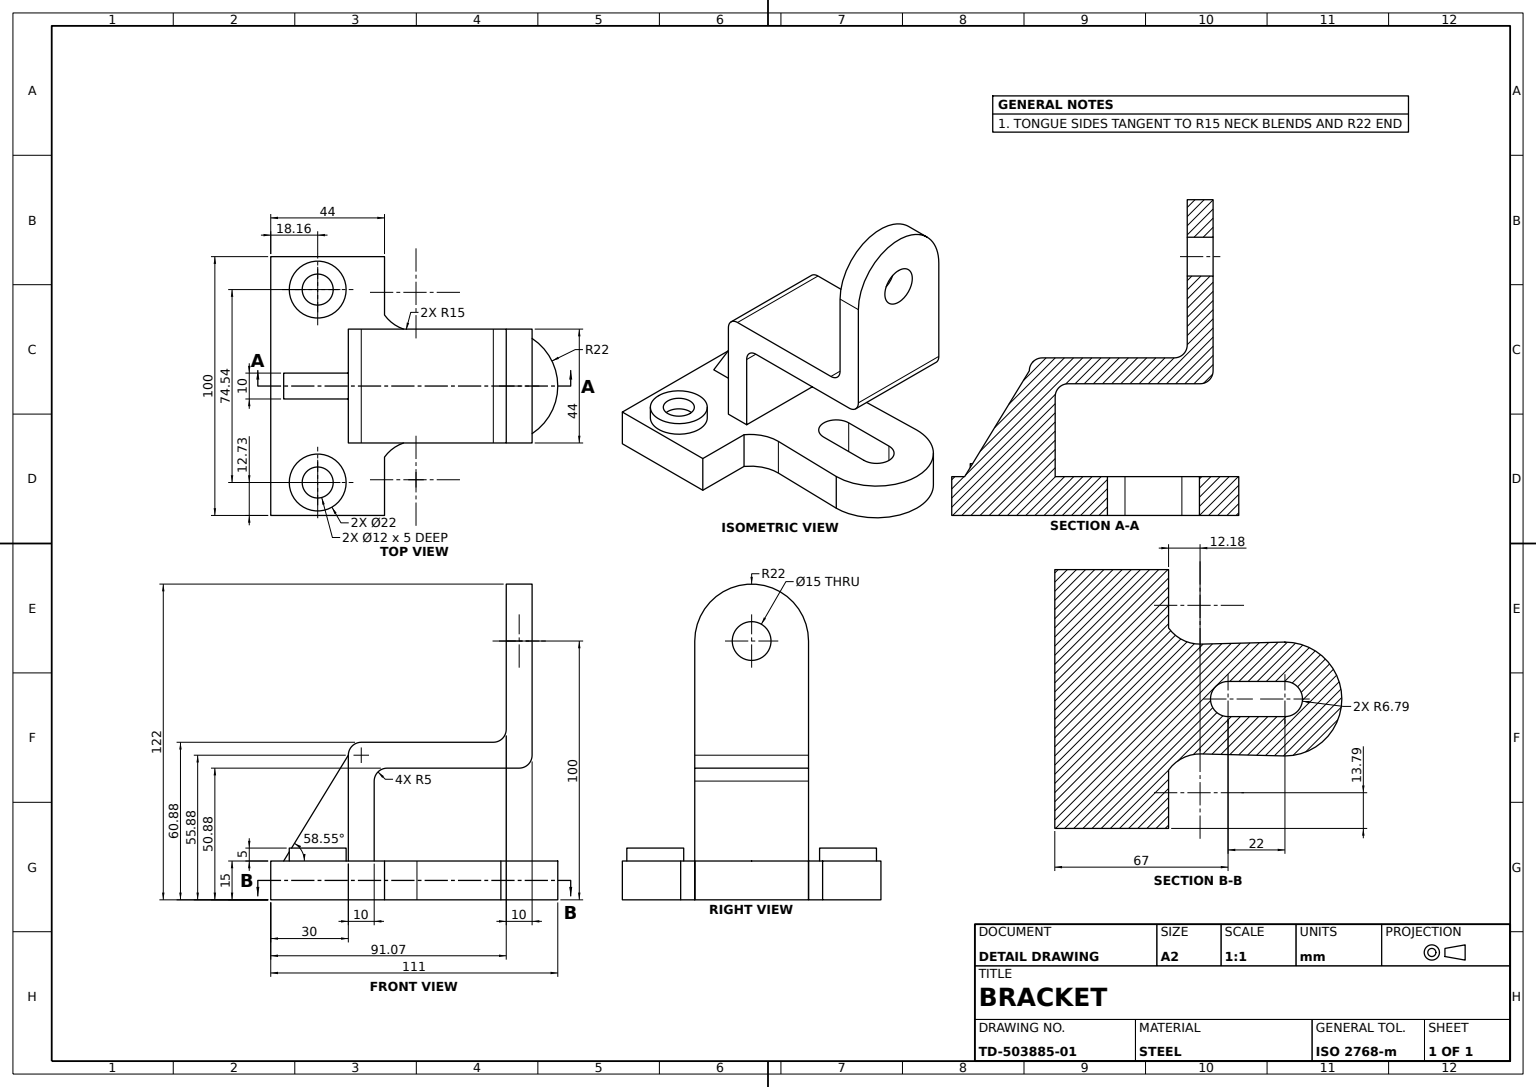
ISO-10303-21;
HEADER;
FILE_DESCRIPTION((''),'2;1');
FILE_NAME('','',(''),(''),'','','');
FILE_SCHEMA(('AUTOMOTIVE_DESIGN'));
ENDSEC;
DATA;
#1=APPLICATION_CONTEXT('');
#2=PRODUCT_CONTEXT('',#1,'mechanical');
#3=PRODUCT('','','',(#2));
#4=PRODUCT_DEFINITION_FORMATION('','',#3);
#5=PRODUCT_DEFINITION_CONTEXT('',#1,'design');
#6=PRODUCT_DEFINITION('','',#4,#5);
#7=PRODUCT_DEFINITION_SHAPE('','',#6);
#8=(LENGTH_UNIT()NAMED_UNIT(*)SI_UNIT(.MILLI.,.METRE.));
#9=(NAMED_UNIT(*)PLANE_ANGLE_UNIT()SI_UNIT($,.RADIAN.));
#10=(NAMED_UNIT(*)SI_UNIT($,.STERADIAN.)SOLID_ANGLE_UNIT());
#11=UNCERTAINTY_MEASURE_WITH_UNIT(LENGTH_MEASURE(1.E-05),#8,'distance_accuracy_value','');
#12=(GEOMETRIC_REPRESENTATION_CONTEXT(3)GLOBAL_UNCERTAINTY_ASSIGNED_CONTEXT((#11))GLOBAL_UNIT_ASSIGNED_CONTEXT((#8,#9,#10))REPRESENTATION_CONTEXT('',''));
#13=CARTESIAN_POINT('',(-9.8432,12.5,-37.27133));
#14=VERTEX_POINT('',#13);
#15=CARTESIAN_POINT('',(2.1568,12.5,-37.27133));
#16=VERTEX_POINT('',#15);
#17=CARTESIAN_POINT('',(-3.8432,12.5,-37.27133));
#18=DIRECTION('',(0.,1.,0.));
#19=DIRECTION('',(-1.,0.,0.));
#20=AXIS2_PLACEMENT_3D('',#17,#18,#19);
#21=CIRCLE('',#20,6.);
#22=EDGE_CURVE('',#14,#16,#21,.T.);
#23=ORIENTED_EDGE('',*,*,#22,.T.);
#24=CARTESIAN_POINT('',(2.1568,7.5,-37.27133));
#25=VERTEX_POINT('',#24);
#26=DIRECTION('',(0.,-1.,0.));
#27=VECTOR('',#26,1000.);
#28=LINE('',#15,#27);
#29=EDGE_CURVE('',#16,#25,#28,.T.);
#30=ORIENTED_EDGE('',*,*,#29,.T.);
#31=CARTESIAN_POINT('',(-9.8432,7.5,-37.27133));
#32=VERTEX_POINT('',#31);
#33=CARTESIAN_POINT('',(-3.8432,7.5,-37.27133));
#34=AXIS2_PLACEMENT_3D('',#33,#18,#19);
#35=CIRCLE('',#34,6.);
#36=EDGE_CURVE('',#32,#25,#35,.T.);
#37=ORIENTED_EDGE('',*,*,#36,.F.);
#38=LINE('',#13,#27);
#39=EDGE_CURVE('',#14,#32,#38,.T.);
#40=ORIENTED_EDGE('',*,*,#39,.F.);
#41=EDGE_LOOP('',(#23,#30,#37,#40));
#42=FACE_OUTER_BOUND('',#41,.T.);
#43=DIRECTION('',(1.,0.,0.));
#44=AXIS2_PLACEMENT_3D('',#17,#26,#43);
#45=CYLINDRICAL_SURFACE('',#44,6.);
#46=ADVANCED_FACE('',(#42),#45,.F.);
#47=CARTESIAN_POINT('',(8.,48.383153,5.));
#48=VERTEX_POINT('',#47);
#49=CARTESIAN_POINT('',(-17.,7.5,5.));
#50=VERTEX_POINT('',#49);
#51=DIRECTION('',(-0.521690821,-0.853134625,0.));
#52=VECTOR('',#51,1000.);
#53=LINE('',#47,#52);
#54=EDGE_CURVE('',#48,#50,#53,.T.);
#55=ORIENTED_EDGE('',*,*,#54,.F.);
#56=CARTESIAN_POINT('',(8.,48.383153,-5.));
#57=VERTEX_POINT('',#56);
#58=DIRECTION('',(0.,0.,-1.));
#59=VECTOR('',#58,1000.);
#60=LINE('',#47,#59);
#61=EDGE_CURVE('',#48,#57,#60,.T.);
#62=ORIENTED_EDGE('',*,*,#61,.T.);
#63=CARTESIAN_POINT('',(-17.,7.5,-5.));
#64=VERTEX_POINT('',#63);
#65=LINE('',#56,#52);
#66=EDGE_CURVE('',#57,#64,#65,.T.);
#67=ORIENTED_EDGE('',*,*,#66,.T.);
#68=LINE('',#49,#59);
#69=EDGE_CURVE('',#50,#64,#68,.T.);
#70=ORIENTED_EDGE('',*,*,#69,.F.);
#71=EDGE_LOOP('',(#55,#62,#67,#70));
#72=FACE_OUTER_BOUND('',#71,.T.);
#73=DIRECTION('',(0.853134625,-0.521690821,0.));
#74=DIRECTION('',(0.521690821,0.853134625,0.));
#75=AXIS2_PLACEMENT_3D('',#47,#73,#74);
#76=PLANE('',#75);
#77=ADVANCED_FACE('',(#72),#76,.F.);
#78=CARTESIAN_POINT('',(34.54142,7.5,-21.210573));
#79=VERTEX_POINT('',#78);
#80=CARTESIAN_POINT('',(34.54142,-7.5,-21.210573));
#81=VERTEX_POINT('',#80);
#82=CARTESIAN_POINT('',(34.54142,94.115575,-21.210573));
#83=LINE('',#82,#27);
#84=EDGE_CURVE('',#79,#81,#83,.T.);
#85=ORIENTED_EDGE('',*,*,#84,.F.);
#86=CARTESIAN_POINT('',(66.991804,7.5,-21.999998));
#87=VERTEX_POINT('',#86);
#88=CARTESIAN_POINT('',(-0.495258,7.5,-20.35823));
#89=DIRECTION('',(-0.999704226,0.,0.024319965));
#90=VECTOR('',#89,1000.);
#91=LINE('',#88,#90);
#92=EDGE_CURVE('',#87,#79,#91,.T.);
#93=ORIENTED_EDGE('',*,*,#92,.F.);
#94=CARTESIAN_POINT('',(66.991804,-7.5,-21.999998));
#95=VERTEX_POINT('',#94);
#96=CARTESIAN_POINT('',(66.991804,94.115575,-21.999998));
#97=LINE('',#96,#27);
#98=EDGE_CURVE('',#87,#95,#97,.T.);
#99=ORIENTED_EDGE('',*,*,#98,.T.);
#100=CARTESIAN_POINT('',(-0.495258,-7.5,-20.35823));
#101=DIRECTION('',(0.999704226,0.,-0.024319965));
#102=VECTOR('',#101,1000.);
#103=LINE('',#100,#102);
#104=EDGE_CURVE('',#81,#95,#103,.T.);
#105=ORIENTED_EDGE('',*,*,#104,.F.);
#106=EDGE_LOOP('',(#85,#93,#99,#105));
#107=FACE_OUTER_BOUND('',#106,.T.);
#108=CARTESIAN_POINT('',(-0.495258,94.115575,-20.35823));
#109=DIRECTION('',(-0.024319965,0.,-0.999704226));
#110=AXIS2_PLACEMENT_3D('',#108,#109,#89);
#111=PLANE('',#110);
#112=ADVANCED_FACE('',(#107),#111,.T.);
#113=CARTESIAN_POINT('',(18.,38.383153,22.));
#114=VERTEX_POINT('',#113);
#115=CARTESIAN_POINT('',(18.,38.383153,-22.));
#116=VERTEX_POINT('',#115);
#117=LINE('',#113,#59);
#118=EDGE_CURVE('',#114,#116,#117,.T.);
#119=ORIENTED_EDGE('',*,*,#118,.F.);
#120=CARTESIAN_POINT('',(18.,7.5,22.));
#121=VERTEX_POINT('',#120);
#122=CARTESIAN_POINT('',(18.,0.,22.));
#123=LINE('',#122,#27);
#124=EDGE_CURVE('',#114,#121,#123,.T.);
#125=ORIENTED_EDGE('',*,*,#124,.T.);
#126=CARTESIAN_POINT('',(18.,7.5,-22.));
#127=VERTEX_POINT('',#126);
#128=LINE('',#120,#59);
#129=EDGE_CURVE('',#121,#127,#128,.T.);
#130=ORIENTED_EDGE('',*,*,#129,.T.);
#131=CARTESIAN_POINT('',(18.,0.,-22.));
#132=LINE('',#131,#27);
#133=EDGE_CURVE('',#116,#127,#132,.T.);
#134=ORIENTED_EDGE('',*,*,#133,.F.);
#135=EDGE_LOOP('',(#119,#125,#130,#134));
#136=FACE_OUTER_BOUND('',#135,.T.);
#137=AXIS2_PLACEMENT_3D('',#122,#43,#18);
#138=PLANE('',#137);
#139=ADVANCED_FACE('',(#136),#138,.T.);
#140=CARTESIAN_POINT('',(73.793313,7.5,0.));
#141=VERTEX_POINT('',#140);
#142=CARTESIAN_POINT('',(67.,7.5,-6.793313));
#143=VERTEX_POINT('',#142);
#144=CARTESIAN_POINT('',(67.,7.5,0.));
#145=AXIS2_PLACEMENT_3D('',#144,#18,#43);
#146=CIRCLE('',#145,6.793313);
#147=EDGE_CURVE('',#141,#143,#146,.T.);
#148=ORIENTED_EDGE('',*,*,#147,.T.);
#149=CARTESIAN_POINT('',(67.,-7.5,-6.793313));
#150=VERTEX_POINT('',#149);
#151=CARTESIAN_POINT('',(67.,94.115575,-6.793313));
#152=LINE('',#151,#27);
#153=EDGE_CURVE('',#143,#150,#152,.T.);
#154=ORIENTED_EDGE('',*,*,#153,.T.);
#155=CARTESIAN_POINT('',(73.793313,-7.5,0.));
#156=VERTEX_POINT('',#155);
#157=CARTESIAN_POINT('',(67.,-7.5,0.));
#158=AXIS2_PLACEMENT_3D('',#157,#26,#43);
#159=CIRCLE('',#158,6.793313);
#160=EDGE_CURVE('',#150,#156,#159,.T.);
#161=ORIENTED_EDGE('',*,*,#160,.T.);
#162=CARTESIAN_POINT('',(73.793313,94.115575,0.));
#163=LINE('',#162,#27);
#164=EDGE_CURVE('',#141,#156,#163,.T.);
#165=ORIENTED_EDGE('',*,*,#164,.F.);
#166=EDGE_LOOP('',(#148,#154,#161,#165));
#167=FACE_OUTER_BOUND('',#166,.T.);
#168=CARTESIAN_POINT('',(67.,94.115575,0.));
#169=AXIS2_PLACEMENT_3D('',#168,#26,#43);
#170=CYLINDRICAL_SURFACE('',#169,6.793313);
#171=ADVANCED_FACE('',(#167),#170,.F.);
#172=ORIENTED_EDGE('',*,*,#66,.F.);
#173=CARTESIAN_POINT('',(8.,7.5,-5.));
#174=VERTEX_POINT('',#173);
#175=VECTOR('',#18,1000.);
#176=LINE('',#173,#175);
#177=EDGE_CURVE('',#174,#57,#176,.T.);
#178=ORIENTED_EDGE('',*,*,#177,.F.);
#179=VECTOR('',#43,1000.);
#180=LINE('',#63,#179);
#181=EDGE_CURVE('',#64,#174,#180,.T.);
#182=ORIENTED_EDGE('',*,*,#181,.F.);
#183=EDGE_LOOP('',(#172,#178,#182));
#184=FACE_OUTER_BOUND('',#183,.T.);
#185=CARTESIAN_POINT('',(0.,0.,-5.));
#186=AXIS2_PLACEMENT_3D('',#185,#58,#19);
#187=PLANE('',#186);
#188=ADVANCED_FACE('',(#184),#187,.T.);
#189=ORIENTED_EDGE('',*,*,#164,.T.);
#190=CARTESIAN_POINT('',(67.,-7.5,6.793313));
#191=VERTEX_POINT('',#190);
#192=EDGE_CURVE('',#156,#191,#159,.T.);
#193=ORIENTED_EDGE('',*,*,#192,.T.);
#194=CARTESIAN_POINT('',(67.,7.5,6.793313));
#195=VERTEX_POINT('',#194);
#196=CARTESIAN_POINT('',(67.,94.115575,6.793313));
#197=LINE('',#196,#27);
#198=EDGE_CURVE('',#195,#191,#197,.T.);
#199=ORIENTED_EDGE('',*,*,#198,.F.);
#200=EDGE_CURVE('',#195,#141,#146,.T.);
#201=ORIENTED_EDGE('',*,*,#200,.T.);
#202=EDGE_LOOP('',(#189,#193,#199,#201));
#203=FACE_OUTER_BOUND('',#202,.T.);
#204=ADVANCED_FACE('',(#203),#170,.F.);
#205=CARTESIAN_POINT('',(8.,7.5,5.));
#206=VERTEX_POINT('',#205);
#207=LINE('',#205,#175);
#208=EDGE_CURVE('',#206,#48,#207,.T.);
#209=ORIENTED_EDGE('',*,*,#208,.F.);
#210=CARTESIAN_POINT('',(8.,7.5,22.));
#211=VERTEX_POINT('',#210);
#212=LINE('',#210,#59);
#213=EDGE_CURVE('',#211,#206,#212,.T.);
#214=ORIENTED_EDGE('',*,*,#213,.F.);
#215=CARTESIAN_POINT('',(8.,48.383153,22.));
#216=VERTEX_POINT('',#215);
#217=CARTESIAN_POINT('',(8.,0.,22.));
#218=LINE('',#217,#175);
#219=EDGE_CURVE('',#211,#216,#218,.T.);
#220=ORIENTED_EDGE('',*,*,#219,.T.);
#221=LINE('',#215,#59);
#222=EDGE_CURVE('',#216,#48,#221,.T.);
#223=ORIENTED_EDGE('',*,*,#222,.T.);
#224=EDGE_LOOP('',(#209,#214,#220,#223));
#225=FACE_OUTER_BOUND('',#224,.T.);
#226=DIRECTION('',(0.,0.,1.));
#227=AXIS2_PLACEMENT_3D('',#217,#19,#226);
#228=PLANE('',#227);
#229=ADVANCED_FACE('',(#225),#228,.T.);
#230=CARTESIAN_POINT('',(-22.,7.5,50.));
#231=VERTEX_POINT('',#230);
#232=CARTESIAN_POINT('',(-22.,-7.5,50.));
#233=VERTEX_POINT('',#232);
#234=CARTESIAN_POINT('',(-22.,0.,50.));
#235=LINE('',#234,#27);
#236=EDGE_CURVE('',#231,#233,#235,.T.);
#237=ORIENTED_EDGE('',*,*,#236,.F.);
#238=CARTESIAN_POINT('',(-22.,7.5,-50.));
#239=VERTEX_POINT('',#238);
#240=LINE('',#230,#59);
#241=EDGE_CURVE('',#231,#239,#240,.T.);
#242=ORIENTED_EDGE('',*,*,#241,.T.);
#243=CARTESIAN_POINT('',(-22.,-7.5,-50.));
#244=VERTEX_POINT('',#243);
#245=CARTESIAN_POINT('',(-22.,0.,-50.));
#246=LINE('',#245,#27);
#247=EDGE_CURVE('',#239,#244,#246,.T.);
#248=ORIENTED_EDGE('',*,*,#247,.T.);
#249=LINE('',#232,#59);
#250=EDGE_CURVE('',#233,#244,#249,.T.);
#251=ORIENTED_EDGE('',*,*,#250,.F.);
#252=EDGE_LOOP('',(#237,#242,#248,#251));
#253=FACE_OUTER_BOUND('',#252,.T.);
#254=AXIS2_PLACEMENT_3D('',#234,#43,#58);
#255=PLANE('',#254);
#256=ADVANCED_FACE('',(#253),#255,.F.);
#257=CARTESIAN_POINT('',(7.1568,12.5,37.27133));
#258=VERTEX_POINT('',#257);
#259=CARTESIAN_POINT('',(7.1568,7.5,37.27133));
#260=VERTEX_POINT('',#259);
#261=LINE('',#257,#27);
#262=EDGE_CURVE('',#258,#260,#261,.T.);
#263=ORIENTED_EDGE('',*,*,#262,.F.);
#264=CARTESIAN_POINT('',(-14.8432,12.5,37.27133));
#265=VERTEX_POINT('',#264);
#266=CARTESIAN_POINT('',(-3.8432,12.5,37.27133));
#267=AXIS2_PLACEMENT_3D('',#266,#18,#43);
#268=CIRCLE('',#267,11.);
#269=EDGE_CURVE('',#265,#258,#268,.T.);
#270=ORIENTED_EDGE('',*,*,#269,.F.);
#271=CARTESIAN_POINT('',(-14.8432,7.5,37.27133));
#272=VERTEX_POINT('',#271);
#273=LINE('',#264,#27);
#274=EDGE_CURVE('',#265,#272,#273,.T.);
#275=ORIENTED_EDGE('',*,*,#274,.T.);
#276=CARTESIAN_POINT('',(-3.8432,7.5,37.27133));
#277=AXIS2_PLACEMENT_3D('',#276,#18,#43);
#278=CIRCLE('',#277,11.);
#279=EDGE_CURVE('',#272,#260,#278,.T.);
#280=ORIENTED_EDGE('',*,*,#279,.T.);
#281=EDGE_LOOP('',(#263,#270,#275,#280));
#282=FACE_OUTER_BOUND('',#281,.T.);
#283=AXIS2_PLACEMENT_3D('',#266,#26,#43);
#284=CYLINDRICAL_SURFACE('',#283,11.);
#285=ADVANCED_FACE('',(#282),#284,.T.);
#286=CARTESIAN_POINT('',(22.,-7.5,-27.446574));
#287=VERTEX_POINT('',#286);
#288=CARTESIAN_POINT('',(34.17662,-7.5,-36.206136));
#289=AXIS2_PLACEMENT_3D('',#288,#18,#43);
#290=CIRCLE('',#289,15.);
#291=EDGE_CURVE('',#287,#81,#290,.T.);
#292=ORIENTED_EDGE('',*,*,#291,.F.);
#293=CARTESIAN_POINT('',(22.,7.5,-27.446574));
#294=VERTEX_POINT('',#293);
#295=CARTESIAN_POINT('',(22.,94.115575,-27.446574));
#296=LINE('',#295,#27);
#297=EDGE_CURVE('',#294,#287,#296,.T.);
#298=ORIENTED_EDGE('',*,*,#297,.F.);
#299=CARTESIAN_POINT('',(34.17662,7.5,-36.206136));
#300=AXIS2_PLACEMENT_3D('',#299,#26,#43);
#301=CIRCLE('',#300,15.);
#302=EDGE_CURVE('',#79,#294,#301,.T.);
#303=ORIENTED_EDGE('',*,*,#302,.F.);
#304=ORIENTED_EDGE('',*,*,#84,.T.);
#305=EDGE_LOOP('',(#292,#298,#303,#304));
#306=FACE_OUTER_BOUND('',#305,.T.);
#307=CARTESIAN_POINT('',(34.17662,94.115575,-36.206136));
#308=AXIS2_PLACEMENT_3D('',#307,#26,#43);
#309=CYLINDRICAL_SURFACE('',#308,15.);
#310=ADVANCED_FACE('',(#306),#309,.F.);
#311=CARTESIAN_POINT('',(64.071732,53.383153,-22.));
#312=VERTEX_POINT('',#311);
#313=CARTESIAN_POINT('',(69.071732,58.383153,-22.));
#314=VERTEX_POINT('',#313);
#315=CARTESIAN_POINT('',(64.071732,58.383153,-22.));
#316=AXIS2_PLACEMENT_3D('',#315,#226,#43);
#317=CIRCLE('',#316,5.);
#318=EDGE_CURVE('',#312,#314,#317,.T.);
#319=ORIENTED_EDGE('',*,*,#318,.F.);
#320=CARTESIAN_POINT('',(64.071732,53.383153,22.));
#321=VERTEX_POINT('',#320);
#322=LINE('',#320,#59);
#323=EDGE_CURVE('',#321,#312,#322,.T.);
#324=ORIENTED_EDGE('',*,*,#323,.F.);
#325=CARTESIAN_POINT('',(69.071732,58.383153,22.));
#326=VERTEX_POINT('',#325);
#327=CARTESIAN_POINT('',(64.071732,58.383153,22.));
#328=AXIS2_PLACEMENT_3D('',#327,#226,#43);
#329=CIRCLE('',#328,5.);
#330=EDGE_CURVE('',#321,#326,#329,.T.);
#331=ORIENTED_EDGE('',*,*,#330,.T.);
#332=LINE('',#325,#59);
#333=EDGE_CURVE('',#326,#314,#332,.T.);
#334=ORIENTED_EDGE('',*,*,#333,.T.);
#335=EDGE_LOOP('',(#319,#324,#331,#334));
#336=FACE_OUTER_BOUND('',#335,.T.);
#337=AXIS2_PLACEMENT_3D('',#327,#58,#19);
#338=CYLINDRICAL_SURFACE('',#337,5.);
#339=ADVANCED_FACE('',(#336),#338,.F.);
#340=ORIENTED_EDGE('',*,*,#274,.F.);
#341=EDGE_CURVE('',#258,#265,#268,.T.);
#342=ORIENTED_EDGE('',*,*,#341,.F.);
#343=ORIENTED_EDGE('',*,*,#262,.T.);
#344=EDGE_CURVE('',#260,#272,#278,.T.);
#345=ORIENTED_EDGE('',*,*,#344,.T.);
#346=EDGE_LOOP('',(#340,#342,#343,#345));
#347=FACE_OUTER_BOUND('',#346,.T.);
#348=ADVANCED_FACE('',(#347),#284,.T.);
#349=CARTESIAN_POINT('',(-14.8432,7.5,-37.27133));
#350=VERTEX_POINT('',#349);
#351=CARTESIAN_POINT('',(7.1568,7.5,-37.27133));
#352=VERTEX_POINT('',#351);
#353=AXIS2_PLACEMENT_3D('',#33,#18,#43);
#354=CIRCLE('',#353,11.);
#355=EDGE_CURVE('',#350,#352,#354,.T.);
#356=ORIENTED_EDGE('',*,*,#355,.T.);
#357=CARTESIAN_POINT('',(7.1568,12.5,-37.27133));
#358=VERTEX_POINT('',#357);
#359=LINE('',#357,#27);
#360=EDGE_CURVE('',#358,#352,#359,.T.);
#361=ORIENTED_EDGE('',*,*,#360,.F.);
#362=CARTESIAN_POINT('',(-14.8432,12.5,-37.27133));
#363=VERTEX_POINT('',#362);
#364=CIRCLE('',#20,11.);
#365=EDGE_CURVE('',#363,#358,#364,.T.);
#366=ORIENTED_EDGE('',*,*,#365,.F.);
#367=LINE('',#362,#27);
#368=EDGE_CURVE('',#363,#350,#367,.T.);
#369=ORIENTED_EDGE('',*,*,#368,.T.);
#370=EDGE_LOOP('',(#356,#361,#366,#369));
#371=FACE_OUTER_BOUND('',#370,.T.);
#372=CYLINDRICAL_SURFACE('',#44,11.);
#373=ADVANCED_FACE('',(#371),#372,.T.);
#374=CARTESIAN_POINT('',(89.,7.5,0.));
#375=VERTEX_POINT('',#374);
#376=CIRCLE('',#145,22.);
#377=EDGE_CURVE('',#375,#87,#376,.T.);
#378=ORIENTED_EDGE('',*,*,#377,.F.);
#379=CARTESIAN_POINT('',(89.,-7.5,0.));
#380=VERTEX_POINT('',#379);
#381=CARTESIAN_POINT('',(89.,94.115575,0.));
#382=LINE('',#381,#27);
#383=EDGE_CURVE('',#375,#380,#382,.T.);
#384=ORIENTED_EDGE('',*,*,#383,.T.);
#385=CIRCLE('',#158,22.);
#386=EDGE_CURVE('',#95,#380,#385,.T.);
#387=ORIENTED_EDGE('',*,*,#386,.F.);
#388=ORIENTED_EDGE('',*,*,#98,.F.);
#389=EDGE_LOOP('',(#378,#384,#387,#388));
#390=FACE_OUTER_BOUND('',#389,.T.);
#391=CYLINDRICAL_SURFACE('',#169,22.);
#392=ADVANCED_FACE('',(#390),#391,.T.);
#393=EDGE_CURVE('',#352,#350,#354,.T.);
#394=ORIENTED_EDGE('',*,*,#393,.T.);
#395=ORIENTED_EDGE('',*,*,#368,.F.);
#396=EDGE_CURVE('',#358,#363,#364,.T.);
#397=ORIENTED_EDGE('',*,*,#396,.F.);
#398=ORIENTED_EDGE('',*,*,#360,.T.);
#399=EDGE_LOOP('',(#394,#395,#397,#398));
#400=FACE_OUTER_BOUND('',#399,.T.);
#401=ADVANCED_FACE('',(#400),#372,.T.);
#402=CARTESIAN_POINT('',(23.,43.383153,22.));
#403=VERTEX_POINT('',#402);
#404=CARTESIAN_POINT('',(23.,43.383153,-22.));
#405=VERTEX_POINT('',#404);
#406=LINE('',#402,#59);
#407=EDGE_CURVE('',#403,#405,#406,.T.);
#408=ORIENTED_EDGE('',*,*,#407,.T.);
#409=CARTESIAN_POINT('',(74.071732,43.383153,-22.));
#410=VERTEX_POINT('',#409);
#411=CARTESIAN_POINT('',(0.,43.383153,-22.));
#412=VECTOR('',#19,1000.);
#413=LINE('',#411,#412);
#414=EDGE_CURVE('',#410,#405,#413,.T.);
#415=ORIENTED_EDGE('',*,*,#414,.F.);
#416=CARTESIAN_POINT('',(74.071732,43.383153,22.));
#417=VERTEX_POINT('',#416);
#418=LINE('',#416,#59);
#419=EDGE_CURVE('',#417,#410,#418,.T.);
#420=ORIENTED_EDGE('',*,*,#419,.F.);
#421=CARTESIAN_POINT('',(0.,43.383153,22.));
#422=LINE('',#421,#412);
#423=EDGE_CURVE('',#417,#403,#422,.T.);
#424=ORIENTED_EDGE('',*,*,#423,.T.);
#425=EDGE_LOOP('',(#408,#415,#420,#424));
#426=FACE_OUTER_BOUND('',#425,.T.);
#427=AXIS2_PLACEMENT_3D('',#421,#26,#43);
#428=PLANE('',#427);
#429=ADVANCED_FACE('',(#426),#428,.T.);
#430=ORIENTED_EDGE('',*,*,#302,.T.);
#431=CARTESIAN_POINT('',(22.,7.5,-50.));
#432=VERTEX_POINT('',#431);
#433=CARTESIAN_POINT('',(22.,7.5,50.));
#434=LINE('',#433,#59);
#435=EDGE_CURVE('',#294,#432,#434,.T.);
#436=ORIENTED_EDGE('',*,*,#435,.T.);
#437=CARTESIAN_POINT('',(0.,7.5,-50.));
#438=LINE('',#437,#412);
#439=EDGE_CURVE('',#432,#239,#438,.T.);
#440=ORIENTED_EDGE('',*,*,#439,.T.);
#441=ORIENTED_EDGE('',*,*,#241,.F.);
#442=VERTEX_POINT('',#433);
#443=CARTESIAN_POINT('',(0.,7.5,50.));
#444=LINE('',#443,#412);
#445=EDGE_CURVE('',#442,#231,#444,.T.);
#446=ORIENTED_EDGE('',*,*,#445,.F.);
#447=CARTESIAN_POINT('',(22.,7.5,27.446574));
#448=VERTEX_POINT('',#447);
#449=EDGE_CURVE('',#442,#448,#434,.T.);
#450=ORIENTED_EDGE('',*,*,#449,.T.);
#451=CARTESIAN_POINT('',(34.54142,7.5,21.210573));
#452=VERTEX_POINT('',#451);
#453=CARTESIAN_POINT('',(34.17662,7.5,36.206136));
#454=AXIS2_PLACEMENT_3D('',#453,#18,#43);
#455=CIRCLE('',#454,15.);
#456=EDGE_CURVE('',#452,#448,#455,.T.);
#457=ORIENTED_EDGE('',*,*,#456,.F.);
#458=CARTESIAN_POINT('',(66.991804,7.5,21.999998));
#459=VERTEX_POINT('',#458);
#460=CARTESIAN_POINT('',(-0.495258,7.5,20.35823));
#461=DIRECTION('',(-0.999704226,0.,-0.024319965));
#462=VECTOR('',#461,1000.);
#463=LINE('',#460,#462);
#464=EDGE_CURVE('',#459,#452,#463,.T.);
#465=ORIENTED_EDGE('',*,*,#464,.F.);
#466=EDGE_CURVE('',#459,#375,#376,.T.);
#467=ORIENTED_EDGE('',*,*,#466,.T.);
#468=ORIENTED_EDGE('',*,*,#377,.T.);
#469=ORIENTED_EDGE('',*,*,#92,.T.);
#470=EDGE_LOOP('',(#430,#436,#440,#441,#446,#450,#457,#465,#467,#468,#469));
#471=FACE_OUTER_BOUND('',#470,.T.);
#472=CARTESIAN_POINT('',(45.,7.5,-6.793313));
#473=VERTEX_POINT('',#472);
#474=CARTESIAN_POINT('',(45.,7.5,6.793313));
#475=VERTEX_POINT('',#474);
#476=CARTESIAN_POINT('',(45.,7.5,0.));
#477=AXIS2_PLACEMENT_3D('',#476,#18,#43);
#478=CIRCLE('',#477,6.793313);
#479=EDGE_CURVE('',#473,#475,#478,.T.);
#480=ORIENTED_EDGE('',*,*,#479,.F.);
#481=CARTESIAN_POINT('',(0.,7.5,-6.793313));
#482=LINE('',#481,#179);
#483=EDGE_CURVE('',#473,#143,#482,.T.);
#484=ORIENTED_EDGE('',*,*,#483,.T.);
#485=ORIENTED_EDGE('',*,*,#147,.F.);
#486=ORIENTED_EDGE('',*,*,#200,.F.);
#487=CARTESIAN_POINT('',(0.,7.5,6.793313));
#488=LINE('',#487,#179);
#489=EDGE_CURVE('',#475,#195,#488,.T.);
#490=ORIENTED_EDGE('',*,*,#489,.F.);
#491=EDGE_LOOP('',(#480,#484,#485,#486,#490));
#492=FACE_BOUND('',#491,.T.);
#493=ORIENTED_EDGE('',*,*,#279,.F.);
#494=ORIENTED_EDGE('',*,*,#344,.F.);
#495=EDGE_LOOP('',(#493,#494));
#496=FACE_BOUND('',#495,.T.);
#497=CARTESIAN_POINT('',(8.,7.5,-22.));
#498=VERTEX_POINT('',#497);
#499=CARTESIAN_POINT('',(0.,7.5,-22.));
#500=LINE('',#499,#412);
#501=EDGE_CURVE('',#127,#498,#500,.T.);
#502=ORIENTED_EDGE('',*,*,#501,.F.);
#503=ORIENTED_EDGE('',*,*,#129,.F.);
#504=CARTESIAN_POINT('',(0.,7.5,22.));
#505=LINE('',#504,#412);
#506=EDGE_CURVE('',#121,#211,#505,.T.);
#507=ORIENTED_EDGE('',*,*,#506,.T.);
#508=ORIENTED_EDGE('',*,*,#213,.T.);
#509=LINE('',#49,#179);
#510=EDGE_CURVE('',#50,#206,#509,.T.);
#511=ORIENTED_EDGE('',*,*,#510,.F.);
#512=ORIENTED_EDGE('',*,*,#69,.T.);
#513=ORIENTED_EDGE('',*,*,#181,.T.);
#514=EDGE_CURVE('',#174,#498,#212,.T.);
#515=ORIENTED_EDGE('',*,*,#514,.T.);
#516=EDGE_LOOP('',(#502,#503,#507,#508,#511,#512,#513,#515));
#517=FACE_BOUND('',#516,.T.);
#518=ORIENTED_EDGE('',*,*,#355,.F.);
#519=ORIENTED_EDGE('',*,*,#393,.F.);
#520=EDGE_LOOP('',(#518,#519));
#521=FACE_BOUND('',#520,.T.);
#522=AXIS2_PLACEMENT_3D('',#443,#26,#43);
#523=PLANE('',#522);
#524=ADVANCED_FACE('',(#471,#492,#496,#517,#521),#523,.F.);
#525=CARTESIAN_POINT('',(-9.8432,7.5,37.27133));
#526=VERTEX_POINT('',#525);
#527=CARTESIAN_POINT('',(2.1568,7.5,37.27133));
#528=VERTEX_POINT('',#527);
#529=CIRCLE('',#277,6.);
#530=EDGE_CURVE('',#526,#528,#529,.T.);
#531=ORIENTED_EDGE('',*,*,#530,.F.);
#532=CARTESIAN_POINT('',(-9.8432,12.5,37.27133));
#533=VERTEX_POINT('',#532);
#534=LINE('',#532,#27);
#535=EDGE_CURVE('',#533,#526,#534,.T.);
#536=ORIENTED_EDGE('',*,*,#535,.F.);
#537=CARTESIAN_POINT('',(2.1568,12.5,37.27133));
#538=VERTEX_POINT('',#537);
#539=CIRCLE('',#267,6.);
#540=EDGE_CURVE('',#533,#538,#539,.T.);
#541=ORIENTED_EDGE('',*,*,#540,.T.);
#542=LINE('',#537,#27);
#543=EDGE_CURVE('',#538,#528,#542,.T.);
#544=ORIENTED_EDGE('',*,*,#543,.T.);
#545=EDGE_LOOP('',(#531,#536,#541,#544));
#546=FACE_OUTER_BOUND('',#545,.T.);
#547=CYLINDRICAL_SURFACE('',#283,6.);
#548=ADVANCED_FACE('',(#546),#547,.F.);
#549=CARTESIAN_POINT('',(69.071732,100.,0.));
#550=VERTEX_POINT('',#549);
#551=CARTESIAN_POINT('',(69.071732,85.,0.));
#552=VERTEX_POINT('',#551);
#553=CARTESIAN_POINT('',(69.071732,92.5,0.));
#554=AXIS2_PLACEMENT_3D('',#553,#19,#26);
#555=CIRCLE('',#554,7.5);
#556=EDGE_CURVE('',#550,#552,#555,.T.);
#557=ORIENTED_EDGE('',*,*,#556,.F.);
#558=EDGE_CURVE('',#552,#550,#555,.T.);
#559=ORIENTED_EDGE('',*,*,#558,.F.);
#560=EDGE_LOOP('',(#557,#559));
#561=FACE_BOUND('',#560,.T.);
#562=CARTESIAN_POINT('',(69.071732,92.5,22.));
#563=VERTEX_POINT('',#562);
#564=CARTESIAN_POINT('',(69.071732,0.,22.));
#565=LINE('',#564,#175);
#566=EDGE_CURVE('',#326,#563,#565,.T.);
#567=ORIENTED_EDGE('',*,*,#566,.T.);
#568=CARTESIAN_POINT('',(69.071732,92.5,-22.));
#569=VERTEX_POINT('',#568);
#570=CIRCLE('',#554,22.);
#571=EDGE_CURVE('',#563,#569,#570,.T.);
#572=ORIENTED_EDGE('',*,*,#571,.T.);
#573=CARTESIAN_POINT('',(69.071732,0.,-22.));
#574=LINE('',#573,#175);
#575=EDGE_CURVE('',#314,#569,#574,.T.);
#576=ORIENTED_EDGE('',*,*,#575,.F.);
#577=ORIENTED_EDGE('',*,*,#333,.F.);
#578=EDGE_LOOP('',(#567,#572,#576,#577));
#579=FACE_OUTER_BOUND('',#578,.T.);
#580=AXIS2_PLACEMENT_3D('',#564,#19,#26);
#581=PLANE('',#580);
#582=ADVANCED_FACE('',(#561,#579),#581,.T.);
#583=ORIENTED_EDGE('',*,*,#396,.T.);
#584=ORIENTED_EDGE('',*,*,#365,.T.);
#585=EDGE_LOOP('',(#583,#584));
#586=FACE_OUTER_BOUND('',#585,.T.);
#587=ORIENTED_EDGE('',*,*,#22,.F.);
#588=EDGE_CURVE('',#16,#14,#21,.T.);
#589=ORIENTED_EDGE('',*,*,#588,.F.);
#590=EDGE_LOOP('',(#587,#589));
#591=FACE_BOUND('',#590,.T.);
#592=PLANE('',#20);
#593=ADVANCED_FACE('',(#586,#591),#592,.T.);
#594=CARTESIAN_POINT('',(45.,-7.5,6.793313));
#595=VERTEX_POINT('',#594);
#596=CARTESIAN_POINT('',(0.,-7.5,6.793313));
#597=LINE('',#596,#412);
#598=EDGE_CURVE('',#191,#595,#597,.T.);
#599=ORIENTED_EDGE('',*,*,#598,.T.);
#600=CARTESIAN_POINT('',(45.,94.115575,6.793313));
#601=LINE('',#600,#27);
#602=EDGE_CURVE('',#475,#595,#601,.T.);
#603=ORIENTED_EDGE('',*,*,#602,.F.);
#604=ORIENTED_EDGE('',*,*,#489,.T.);
#605=ORIENTED_EDGE('',*,*,#198,.T.);
#606=EDGE_LOOP('',(#599,#603,#604,#605));
#607=FACE_OUTER_BOUND('',#606,.T.);
#608=CARTESIAN_POINT('',(0.,94.115575,6.793313));
#609=AXIS2_PLACEMENT_3D('',#608,#226,#43);
#610=PLANE('',#609);
#611=ADVANCED_FACE('',(#607),#610,.F.);
#612=ORIENTED_EDGE('',*,*,#54,.T.);
#613=ORIENTED_EDGE('',*,*,#510,.T.);
#614=ORIENTED_EDGE('',*,*,#208,.T.);
#615=EDGE_LOOP('',(#612,#613,#614));
#616=FACE_OUTER_BOUND('',#615,.T.);
#617=CARTESIAN_POINT('',(0.,0.,5.));
#618=AXIS2_PLACEMENT_3D('',#617,#58,#19);
#619=PLANE('',#618);
#620=ADVANCED_FACE('',(#616),#619,.F.);
#621=CARTESIAN_POINT('',(13.,53.383153,22.));
#622=VERTEX_POINT('',#621);
#623=CARTESIAN_POINT('',(0.,53.383153,22.));
#624=LINE('',#623,#179);
#625=EDGE_CURVE('',#622,#321,#624,.T.);
#626=ORIENTED_EDGE('',*,*,#625,.F.);
#627=CARTESIAN_POINT('',(13.,48.383153,22.));
#628=AXIS2_PLACEMENT_3D('',#627,#58,#43);
#629=CIRCLE('',#628,5.);
#630=EDGE_CURVE('',#216,#622,#629,.T.);
#631=ORIENTED_EDGE('',*,*,#630,.F.);
#632=ORIENTED_EDGE('',*,*,#219,.F.);
#633=ORIENTED_EDGE('',*,*,#506,.F.);
#634=ORIENTED_EDGE('',*,*,#124,.F.);
#635=CARTESIAN_POINT('',(23.,38.383153,22.));
#636=AXIS2_PLACEMENT_3D('',#635,#226,#43);
#637=CIRCLE('',#636,5.);
#638=EDGE_CURVE('',#403,#114,#637,.T.);
#639=ORIENTED_EDGE('',*,*,#638,.F.);
#640=ORIENTED_EDGE('',*,*,#423,.F.);
#641=CARTESIAN_POINT('',(79.071732,48.383153,22.));
#642=VERTEX_POINT('',#641);
#643=CARTESIAN_POINT('',(74.071732,48.383153,22.));
#644=AXIS2_PLACEMENT_3D('',#643,#58,#43);
#645=CIRCLE('',#644,5.);
#646=EDGE_CURVE('',#642,#417,#645,.T.);
#647=ORIENTED_EDGE('',*,*,#646,.F.);
#648=CARTESIAN_POINT('',(79.071732,92.5,22.));
#649=VERTEX_POINT('',#648);
#650=CARTESIAN_POINT('',(79.071732,0.,22.));
#651=LINE('',#650,#27);
#652=EDGE_CURVE('',#649,#642,#651,.T.);
#653=ORIENTED_EDGE('',*,*,#652,.F.);
#654=CARTESIAN_POINT('',(0.,92.5,22.));
#655=LINE('',#654,#179);
#656=EDGE_CURVE('',#563,#649,#655,.T.);
#657=ORIENTED_EDGE('',*,*,#656,.F.);
#658=ORIENTED_EDGE('',*,*,#566,.F.);
#659=ORIENTED_EDGE('',*,*,#330,.F.);
#660=EDGE_LOOP('',(#626,#631,#632,#633,#634,#639,#640,#647,#653,#657,#658,#659));
#661=FACE_OUTER_BOUND('',#660,.T.);
#662=CARTESIAN_POINT('',(0.,0.,22.));
#663=AXIS2_PLACEMENT_3D('',#662,#226,#43);
#664=PLANE('',#663);
#665=ADVANCED_FACE('',(#661),#664,.T.);
#666=ORIENTED_EDGE('',*,*,#36,.T.);
#667=EDGE_CURVE('',#25,#32,#35,.T.);
#668=ORIENTED_EDGE('',*,*,#667,.T.);
#669=EDGE_LOOP('',(#666,#668));
#670=FACE_OUTER_BOUND('',#669,.T.);
#671=ADVANCED_FACE('',(#670),#523,.F.);
#672=ORIENTED_EDGE('',*,*,#602,.T.);
#673=CARTESIAN_POINT('',(45.,-7.5,-6.793313));
#674=VERTEX_POINT('',#673);
#675=CARTESIAN_POINT('',(45.,-7.5,0.));
#676=AXIS2_PLACEMENT_3D('',#675,#26,#43);
#677=CIRCLE('',#676,6.793313);
#678=EDGE_CURVE('',#595,#674,#677,.T.);
#679=ORIENTED_EDGE('',*,*,#678,.T.);
#680=CARTESIAN_POINT('',(45.,94.115575,-6.793313));
#681=LINE('',#680,#27);
#682=EDGE_CURVE('',#473,#674,#681,.T.);
#683=ORIENTED_EDGE('',*,*,#682,.F.);
#684=ORIENTED_EDGE('',*,*,#479,.T.);
#685=EDGE_LOOP('',(#672,#679,#683,#684));
#686=FACE_OUTER_BOUND('',#685,.T.);
#687=CARTESIAN_POINT('',(45.,94.115575,0.));
#688=AXIS2_PLACEMENT_3D('',#687,#26,#43);
#689=CYLINDRICAL_SURFACE('',#688,6.793313);
#690=ADVANCED_FACE('',(#686),#689,.F.);
#691=ORIENTED_EDGE('',*,*,#638,.T.);
#692=ORIENTED_EDGE('',*,*,#118,.T.);
#693=CARTESIAN_POINT('',(23.,38.383153,-22.));
#694=AXIS2_PLACEMENT_3D('',#693,#226,#43);
#695=CIRCLE('',#694,5.);
#696=EDGE_CURVE('',#405,#116,#695,.T.);
#697=ORIENTED_EDGE('',*,*,#696,.F.);
#698=ORIENTED_EDGE('',*,*,#407,.F.);
#699=EDGE_LOOP('',(#691,#692,#697,#698));
#700=FACE_OUTER_BOUND('',#699,.T.);
#701=AXIS2_PLACEMENT_3D('',#635,#58,#19);
#702=CYLINDRICAL_SURFACE('',#701,5.);
#703=ADVANCED_FACE('',(#700),#702,.F.);
#704=CARTESIAN_POINT('',(79.071732,48.383153,-22.));
#705=VERTEX_POINT('',#704);
#706=CARTESIAN_POINT('',(74.071732,48.383153,-22.));
#707=AXIS2_PLACEMENT_3D('',#706,#58,#43);
#708=CIRCLE('',#707,5.);
#709=EDGE_CURVE('',#705,#410,#708,.T.);
#710=ORIENTED_EDGE('',*,*,#709,.F.);
#711=LINE('',#641,#59);
#712=EDGE_CURVE('',#642,#705,#711,.T.);
#713=ORIENTED_EDGE('',*,*,#712,.F.);
#714=ORIENTED_EDGE('',*,*,#646,.T.);
#715=ORIENTED_EDGE('',*,*,#419,.T.);
#716=EDGE_LOOP('',(#710,#713,#714,#715));
#717=FACE_OUTER_BOUND('',#716,.T.);
#718=AXIS2_PLACEMENT_3D('',#643,#58,#19);
#719=CYLINDRICAL_SURFACE('',#718,5.);
#720=ADVANCED_FACE('',(#717),#719,.T.);
#721=CARTESIAN_POINT('',(22.,-7.5,27.446574));
#722=VERTEX_POINT('',#721);
#723=CARTESIAN_POINT('',(22.,94.115575,27.446574));
#724=LINE('',#723,#27);
#725=EDGE_CURVE('',#448,#722,#724,.T.);
#726=ORIENTED_EDGE('',*,*,#725,.F.);
#727=ORIENTED_EDGE('',*,*,#449,.F.);
#728=CARTESIAN_POINT('',(22.,-7.5,50.));
#729=VERTEX_POINT('',#728);
#730=CARTESIAN_POINT('',(22.,0.,50.));
#731=LINE('',#730,#27);
#732=EDGE_CURVE('',#442,#729,#731,.T.);
#733=ORIENTED_EDGE('',*,*,#732,.T.);
#734=LINE('',#728,#59);
#735=EDGE_CURVE('',#729,#722,#734,.T.);
#736=ORIENTED_EDGE('',*,*,#735,.T.);
#737=EDGE_LOOP('',(#726,#727,#733,#736));
#738=FACE_OUTER_BOUND('',#737,.T.);
#739=AXIS2_PLACEMENT_3D('',#730,#43,#58);
#740=PLANE('',#739);
#741=ADVANCED_FACE('',(#738),#740,.T.);
#742=ORIENTED_EDGE('',*,*,#29,.F.);
#743=ORIENTED_EDGE('',*,*,#588,.T.);
#744=ORIENTED_EDGE('',*,*,#39,.T.);
#745=ORIENTED_EDGE('',*,*,#667,.F.);
#746=EDGE_LOOP('',(#742,#743,#744,#745));
#747=FACE_OUTER_BOUND('',#746,.T.);
#748=ADVANCED_FACE('',(#747),#45,.F.);
#749=ORIENTED_EDGE('',*,*,#456,.T.);
#750=ORIENTED_EDGE('',*,*,#725,.T.);
#751=CARTESIAN_POINT('',(34.54142,-7.5,21.210573));
#752=VERTEX_POINT('',#751);
#753=CARTESIAN_POINT('',(34.17662,-7.5,36.206136));
#754=AXIS2_PLACEMENT_3D('',#753,#26,#43);
#755=CIRCLE('',#754,15.);
#756=EDGE_CURVE('',#722,#752,#755,.T.);
#757=ORIENTED_EDGE('',*,*,#756,.T.);
#758=CARTESIAN_POINT('',(34.54142,94.115575,21.210573));
#759=LINE('',#758,#27);
#760=EDGE_CURVE('',#452,#752,#759,.T.);
#761=ORIENTED_EDGE('',*,*,#760,.F.);
#762=EDGE_LOOP('',(#749,#750,#757,#761));
#763=FACE_OUTER_BOUND('',#762,.T.);
#764=CARTESIAN_POINT('',(34.17662,94.115575,36.206136));
#765=AXIS2_PLACEMENT_3D('',#764,#26,#43);
#766=CYLINDRICAL_SURFACE('',#765,15.);
#767=ADVANCED_FACE('',(#763),#766,.F.);
#768=ORIENTED_EDGE('',*,*,#656,.T.);
#769=CARTESIAN_POINT('',(79.071732,92.5,-22.));
#770=VERTEX_POINT('',#769);
#771=CARTESIAN_POINT('',(79.071732,92.5,0.));
#772=AXIS2_PLACEMENT_3D('',#771,#19,#58);
#773=CIRCLE('',#772,22.);
#774=EDGE_CURVE('',#649,#770,#773,.T.);
#775=ORIENTED_EDGE('',*,*,#774,.T.);
#776=CARTESIAN_POINT('',(0.,92.5,-22.));
#777=LINE('',#776,#179);
#778=EDGE_CURVE('',#569,#770,#777,.T.);
#779=ORIENTED_EDGE('',*,*,#778,.F.);
#780=ORIENTED_EDGE('',*,*,#571,.F.);
#781=EDGE_LOOP('',(#768,#775,#779,#780));
#782=FACE_OUTER_BOUND('',#781,.T.);
#783=CARTESIAN_POINT('',(128.265227,92.5,0.));
#784=AXIS2_PLACEMENT_3D('',#783,#19,#26);
#785=CYLINDRICAL_SURFACE('',#784,22.);
#786=ADVANCED_FACE('',(#782),#785,.T.);
#787=ORIENTED_EDGE('',*,*,#709,.T.);
#788=ORIENTED_EDGE('',*,*,#414,.T.);
#789=ORIENTED_EDGE('',*,*,#696,.T.);
#790=ORIENTED_EDGE('',*,*,#133,.T.);
#791=ORIENTED_EDGE('',*,*,#501,.T.);
#792=CARTESIAN_POINT('',(8.,48.383153,-22.));
#793=VERTEX_POINT('',#792);
#794=CARTESIAN_POINT('',(8.,0.,-22.));
#795=LINE('',#794,#175);
#796=EDGE_CURVE('',#498,#793,#795,.T.);
#797=ORIENTED_EDGE('',*,*,#796,.T.);
#798=CARTESIAN_POINT('',(13.,53.383153,-22.));
#799=VERTEX_POINT('',#798);
#800=CARTESIAN_POINT('',(13.,48.383153,-22.));
#801=AXIS2_PLACEMENT_3D('',#800,#58,#43);
#802=CIRCLE('',#801,5.);
#803=EDGE_CURVE('',#793,#799,#802,.T.);
#804=ORIENTED_EDGE('',*,*,#803,.T.);
#805=CARTESIAN_POINT('',(0.,53.383153,-22.));
#806=LINE('',#805,#179);
#807=EDGE_CURVE('',#799,#312,#806,.T.);
#808=ORIENTED_EDGE('',*,*,#807,.T.);
#809=ORIENTED_EDGE('',*,*,#318,.T.);
#810=ORIENTED_EDGE('',*,*,#575,.T.);
#811=ORIENTED_EDGE('',*,*,#778,.T.);
#812=CARTESIAN_POINT('',(79.071732,0.,-22.));
#813=LINE('',#812,#27);
#814=EDGE_CURVE('',#770,#705,#813,.T.);
#815=ORIENTED_EDGE('',*,*,#814,.T.);
#816=EDGE_LOOP('',(#787,#788,#789,#790,#791,#797,#804,#808,#809,#810,#811,#815));
#817=FACE_OUTER_BOUND('',#816,.T.);
#818=CARTESIAN_POINT('',(0.,0.,-22.));
#819=AXIS2_PLACEMENT_3D('',#818,#226,#43);
#820=PLANE('',#819);
#821=ADVANCED_FACE('',(#817),#820,.F.);
#822=ORIENTED_EDGE('',*,*,#514,.F.);
#823=ORIENTED_EDGE('',*,*,#177,.T.);
#824=EDGE_CURVE('',#57,#793,#221,.T.);
#825=ORIENTED_EDGE('',*,*,#824,.T.);
#826=ORIENTED_EDGE('',*,*,#796,.F.);
#827=EDGE_LOOP('',(#822,#823,#825,#826));
#828=FACE_OUTER_BOUND('',#827,.T.);
#829=ADVANCED_FACE('',(#828),#228,.T.);
#830=ORIENTED_EDGE('',*,*,#530,.T.);
#831=EDGE_CURVE('',#528,#526,#529,.T.);
#832=ORIENTED_EDGE('',*,*,#831,.T.);
#833=EDGE_LOOP('',(#830,#832));
#834=FACE_OUTER_BOUND('',#833,.T.);
#835=ADVANCED_FACE('',(#834),#523,.F.);
#836=ORIENTED_EDGE('',*,*,#236,.T.);
#837=CARTESIAN_POINT('',(0.,-7.5,50.));
#838=LINE('',#837,#412);
#839=EDGE_CURVE('',#729,#233,#838,.T.);
#840=ORIENTED_EDGE('',*,*,#839,.F.);
#841=ORIENTED_EDGE('',*,*,#732,.F.);
#842=ORIENTED_EDGE('',*,*,#445,.T.);
#843=EDGE_LOOP('',(#836,#840,#841,#842));
#844=FACE_OUTER_BOUND('',#843,.T.);
#845=CARTESIAN_POINT('',(0.,0.,50.));
#846=AXIS2_PLACEMENT_3D('',#845,#226,#43);
#847=PLANE('',#846);
#848=ADVANCED_FACE('',(#844),#847,.T.);
#849=ORIENTED_EDGE('',*,*,#598,.F.);
#850=ORIENTED_EDGE('',*,*,#192,.F.);
#851=ORIENTED_EDGE('',*,*,#160,.F.);
#852=CARTESIAN_POINT('',(0.,-7.5,-6.793313));
#853=LINE('',#852,#412);
#854=EDGE_CURVE('',#150,#674,#853,.T.);
#855=ORIENTED_EDGE('',*,*,#854,.T.);
#856=ORIENTED_EDGE('',*,*,#678,.F.);
#857=EDGE_LOOP('',(#849,#850,#851,#855,#856));
#858=FACE_BOUND('',#857,.T.);
#859=ORIENTED_EDGE('',*,*,#735,.F.);
#860=ORIENTED_EDGE('',*,*,#839,.T.);
#861=ORIENTED_EDGE('',*,*,#250,.T.);
#862=CARTESIAN_POINT('',(22.,-7.5,-50.));
#863=VERTEX_POINT('',#862);
#864=CARTESIAN_POINT('',(0.,-7.5,-50.));
#865=LINE('',#864,#412);
#866=EDGE_CURVE('',#863,#244,#865,.T.);
#867=ORIENTED_EDGE('',*,*,#866,.F.);
#868=EDGE_CURVE('',#287,#863,#734,.T.);
#869=ORIENTED_EDGE('',*,*,#868,.F.);
#870=ORIENTED_EDGE('',*,*,#291,.T.);
#871=ORIENTED_EDGE('',*,*,#104,.T.);
#872=ORIENTED_EDGE('',*,*,#386,.T.);
#873=CARTESIAN_POINT('',(66.991804,-7.5,21.999998));
#874=VERTEX_POINT('',#873);
#875=EDGE_CURVE('',#380,#874,#385,.T.);
#876=ORIENTED_EDGE('',*,*,#875,.T.);
#877=CARTESIAN_POINT('',(-0.495258,-7.5,20.35823));
#878=DIRECTION('',(0.999704226,0.,0.024319965));
#879=VECTOR('',#878,1000.);
#880=LINE('',#877,#879);
#881=EDGE_CURVE('',#752,#874,#880,.T.);
#882=ORIENTED_EDGE('',*,*,#881,.F.);
#883=ORIENTED_EDGE('',*,*,#756,.F.);
#884=EDGE_LOOP('',(#859,#860,#861,#867,#869,#870,#871,#872,#876,#882,#883));
#885=FACE_OUTER_BOUND('',#884,.T.);
#886=AXIS2_PLACEMENT_3D('',#837,#26,#43);
#887=PLANE('',#886);
#888=ADVANCED_FACE('',(#858,#885),#887,.T.);
#889=CARTESIAN_POINT('',(22.,0.,-50.));
#890=LINE('',#889,#27);
#891=EDGE_CURVE('',#432,#863,#890,.T.);
#892=ORIENTED_EDGE('',*,*,#891,.T.);
#893=ORIENTED_EDGE('',*,*,#866,.T.);
#894=ORIENTED_EDGE('',*,*,#247,.F.);
#895=ORIENTED_EDGE('',*,*,#439,.F.);
#896=EDGE_LOOP('',(#892,#893,#894,#895));
#897=FACE_OUTER_BOUND('',#896,.T.);
#898=CARTESIAN_POINT('',(0.,0.,-50.));
#899=AXIS2_PLACEMENT_3D('',#898,#226,#43);
#900=PLANE('',#899);
#901=ADVANCED_FACE('',(#897),#900,.F.);
#902=CARTESIAN_POINT('',(79.071732,85.,0.));
#903=VERTEX_POINT('',#902);
#904=CARTESIAN_POINT('',(128.265227,85.,0.));
#905=LINE('',#904,#412);
#906=EDGE_CURVE('',#903,#552,#905,.T.);
#907=ORIENTED_EDGE('',*,*,#906,.F.);
#908=CARTESIAN_POINT('',(79.071732,100.,0.));
#909=VERTEX_POINT('',#908);
#910=CIRCLE('',#772,7.5);
#911=EDGE_CURVE('',#909,#903,#910,.T.);
#912=ORIENTED_EDGE('',*,*,#911,.F.);
#913=CARTESIAN_POINT('',(128.265227,100.,0.));
#914=LINE('',#913,#412);
#915=EDGE_CURVE('',#909,#550,#914,.T.);
#916=ORIENTED_EDGE('',*,*,#915,.T.);
#917=ORIENTED_EDGE('',*,*,#556,.T.);
#918=EDGE_LOOP('',(#907,#912,#916,#917));
#919=FACE_OUTER_BOUND('',#918,.T.);
#920=CYLINDRICAL_SURFACE('',#784,7.5);
#921=ADVANCED_FACE('',(#919),#920,.F.);
#922=CARTESIAN_POINT('',(66.991804,94.115575,21.999998));
#923=LINE('',#922,#27);
#924=EDGE_CURVE('',#459,#874,#923,.T.);
#925=ORIENTED_EDGE('',*,*,#924,.T.);
#926=ORIENTED_EDGE('',*,*,#875,.F.);
#927=ORIENTED_EDGE('',*,*,#383,.F.);
#928=ORIENTED_EDGE('',*,*,#466,.F.);
#929=EDGE_LOOP('',(#925,#926,#927,#928));
#930=FACE_OUTER_BOUND('',#929,.T.);
#931=ADVANCED_FACE('',(#930),#391,.T.);
#932=ORIENTED_EDGE('',*,*,#807,.F.);
#933=LINE('',#621,#59);
#934=EDGE_CURVE('',#622,#799,#933,.T.);
#935=ORIENTED_EDGE('',*,*,#934,.F.);
#936=ORIENTED_EDGE('',*,*,#625,.T.);
#937=ORIENTED_EDGE('',*,*,#323,.T.);
#938=EDGE_LOOP('',(#932,#935,#936,#937));
#939=FACE_OUTER_BOUND('',#938,.T.);
#940=AXIS2_PLACEMENT_3D('',#623,#18,#226);
#941=PLANE('',#940);
#942=ADVANCED_FACE('',(#939),#941,.T.);
#943=ORIENTED_EDGE('',*,*,#854,.F.);
#944=ORIENTED_EDGE('',*,*,#153,.F.);
#945=ORIENTED_EDGE('',*,*,#483,.F.);
#946=ORIENTED_EDGE('',*,*,#682,.T.);
#947=EDGE_LOOP('',(#943,#944,#945,#946));
#948=FACE_OUTER_BOUND('',#947,.T.);
#949=CARTESIAN_POINT('',(0.,94.115575,-6.793313));
#950=AXIS2_PLACEMENT_3D('',#949,#226,#43);
#951=PLANE('',#950);
#952=ADVANCED_FACE('',(#948),#951,.T.);
#953=ORIENTED_EDGE('',*,*,#803,.F.);
#954=ORIENTED_EDGE('',*,*,#824,.F.);
#955=ORIENTED_EDGE('',*,*,#61,.F.);
#956=ORIENTED_EDGE('',*,*,#222,.F.);
#957=ORIENTED_EDGE('',*,*,#630,.T.);
#958=ORIENTED_EDGE('',*,*,#934,.T.);
#959=EDGE_LOOP('',(#953,#954,#955,#956,#957,#958));
#960=FACE_OUTER_BOUND('',#959,.T.);
#961=AXIS2_PLACEMENT_3D('',#627,#58,#19);
#962=CYLINDRICAL_SURFACE('',#961,5.);
#963=ADVANCED_FACE('',(#960),#962,.T.);
#964=ORIENTED_EDGE('',*,*,#831,.F.);
#965=ORIENTED_EDGE('',*,*,#543,.F.);
#966=EDGE_CURVE('',#538,#533,#539,.T.);
#967=ORIENTED_EDGE('',*,*,#966,.T.);
#968=ORIENTED_EDGE('',*,*,#535,.T.);
#969=EDGE_LOOP('',(#964,#965,#967,#968));
#970=FACE_OUTER_BOUND('',#969,.T.);
#971=ADVANCED_FACE('',(#970),#547,.F.);
#972=ORIENTED_EDGE('',*,*,#911,.T.);
#973=EDGE_CURVE('',#903,#909,#910,.T.);
#974=ORIENTED_EDGE('',*,*,#973,.T.);
#975=EDGE_LOOP('',(#972,#974));
#976=FACE_BOUND('',#975,.T.);
#977=ORIENTED_EDGE('',*,*,#712,.T.);
#978=ORIENTED_EDGE('',*,*,#814,.F.);
#979=ORIENTED_EDGE('',*,*,#774,.F.);
#980=ORIENTED_EDGE('',*,*,#652,.T.);
#981=EDGE_LOOP('',(#977,#978,#979,#980));
#982=FACE_OUTER_BOUND('',#981,.T.);
#983=AXIS2_PLACEMENT_3D('',#650,#43,#58);
#984=PLANE('',#983);
#985=ADVANCED_FACE('',(#976,#982),#984,.T.);
#986=ORIENTED_EDGE('',*,*,#881,.T.);
#987=ORIENTED_EDGE('',*,*,#924,.F.);
#988=ORIENTED_EDGE('',*,*,#464,.T.);
#989=ORIENTED_EDGE('',*,*,#760,.T.);
#990=EDGE_LOOP('',(#986,#987,#988,#989));
#991=FACE_OUTER_BOUND('',#990,.T.);
#992=CARTESIAN_POINT('',(-0.495258,94.115575,20.35823));
#993=DIRECTION('',(0.024319965,0.,-0.999704226));
#994=AXIS2_PLACEMENT_3D('',#992,#993,#461);
#995=PLANE('',#994);
#996=ADVANCED_FACE('',(#991),#995,.F.);
#997=ORIENTED_EDGE('',*,*,#269,.T.);
#998=ORIENTED_EDGE('',*,*,#341,.T.);
#999=EDGE_LOOP('',(#997,#998));
#1000=FACE_OUTER_BOUND('',#999,.T.);
#1001=ORIENTED_EDGE('',*,*,#966,.F.);
#1002=ORIENTED_EDGE('',*,*,#540,.F.);
#1003=EDGE_LOOP('',(#1001,#1002));
#1004=FACE_BOUND('',#1003,.T.);
#1005=PLANE('',#283);
#1006=ADVANCED_FACE('',(#1000,#1004),#1005,.F.);
#1007=ORIENTED_EDGE('',*,*,#973,.F.);
#1008=ORIENTED_EDGE('',*,*,#906,.T.);
#1009=ORIENTED_EDGE('',*,*,#558,.T.);
#1010=ORIENTED_EDGE('',*,*,#915,.F.);
#1011=EDGE_LOOP('',(#1007,#1008,#1009,#1010));
#1012=FACE_OUTER_BOUND('',#1011,.T.);
#1013=ADVANCED_FACE('',(#1012),#920,.F.);
#1014=ORIENTED_EDGE('',*,*,#868,.T.);
#1015=ORIENTED_EDGE('',*,*,#891,.F.);
#1016=ORIENTED_EDGE('',*,*,#435,.F.);
#1017=ORIENTED_EDGE('',*,*,#297,.T.);
#1018=EDGE_LOOP('',(#1014,#1015,#1016,#1017));
#1019=FACE_OUTER_BOUND('',#1018,.T.);
#1020=ADVANCED_FACE('',(#1019),#740,.T.);
#1021=CLOSED_SHELL('',(#46,#77,#112,#139,#171,#188,#204,#229,#256,#285,#310,#339,#348,#373,#392,#401,#429,#524,#548,#582,#593,#611,#620,#665,#671,#690,#703,#720,#741,#748,#767,#786,#821,#829,#835,#848,#888,#901,#921,#931,#942,#952,#963,#971,#985,#996,#1006,#1013,#1020));
#1022=MANIFOLD_SOLID_BREP('',#1021);
#1023=ADVANCED_BREP_SHAPE_REPRESENTATION('',(#1022),#12);
#1024=SHAPE_DEFINITION_REPRESENTATION(#7,#1023);
ENDSEC;
END-ISO-10303-21;
